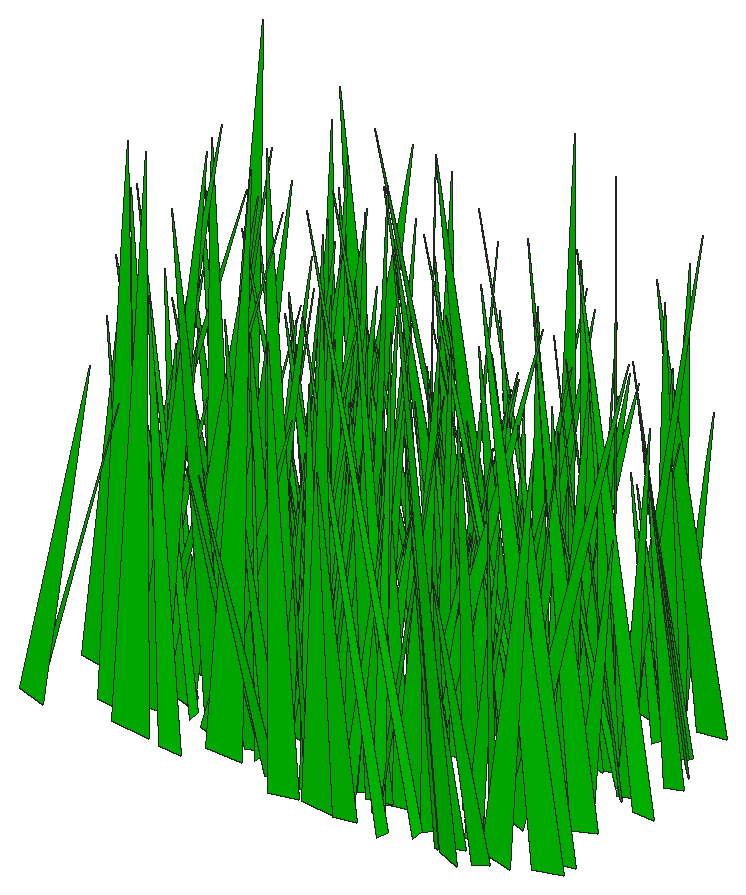
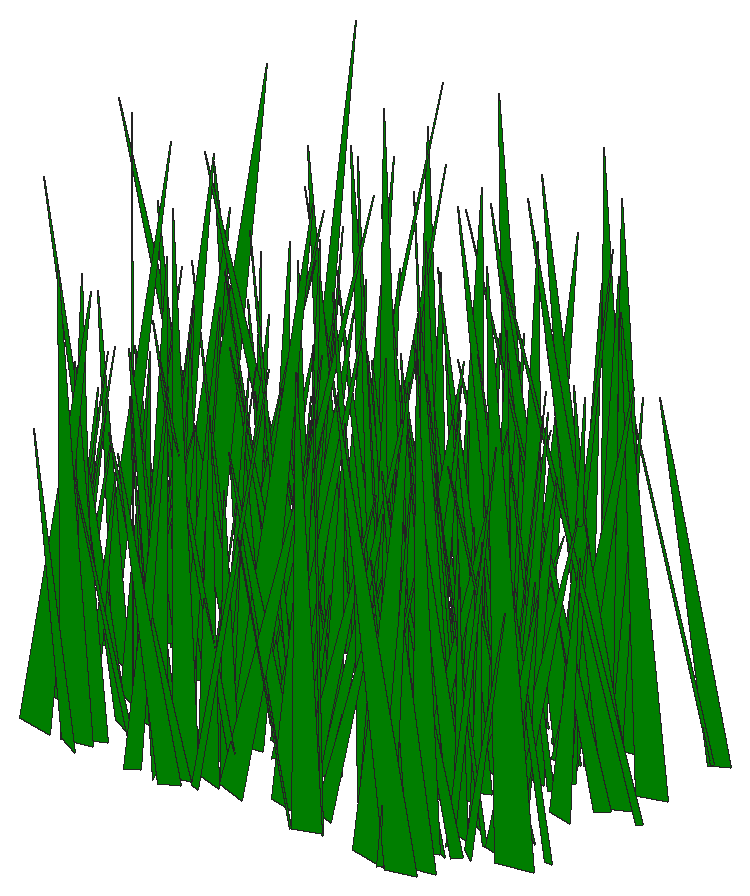
# SketchUp Ruby script. Lengths in inches.
U = 1.inch
M = Sketchup.active_model
def pt(a) = Geom::Point3d.new(a.map { |v| v * U })
def face(e, loops, mat)
  f = e.add_face(loops[0].map { |a| pt(a) })
  loops[1..].each { |l| e.add_face(l.map { |a| pt(a) }).erase! }
  f.material = f.back_material = mat if mat
  f
end
# faces: each face lists its corners as indices into pts; further lists are holes
def faces(e, pts, list, mat = nil) = list.each { |f| face(e, (f[0].is_a?(Array) ? f : [f]).map { |l| l.map { |i| pts[i] } }, mat) }
# xy, xz, yz: faces in a plane at the given z, y or x. An outline is a flat list of corners, or four numbers for a rectangle; further outlines are holes
def ring(l) = l.size == 4 ? [[l[0], l[1]], [l[2], l[1]], [l[2], l[3]], [l[0], l[3]]] : l.each_slice(2).to_a
def flat(e, list, mat, &to3) = list.each { |f| face(e, (f[0].is_a?(Array) ? f : [f]).map { |l| ring(l).map { |u, v| to3.(u, v) } }, mat) }
def xy(e, z, list, mat = nil) = flat(e, list, mat) { |x, y| [x, y, z] }
def xz(e, y, list, mat = nil) = flat(e, list, mat) { |x, z| [x, y, z] }
def yz(e, x, list, mat = nil) = flat(e, list, mat) { |y, z| [x, y, z] }
def lines(e, pts, list) = list.each { |a, b| e.add_line(pt(pts[a]), pt(pts[b])) }
# prism: a flat outline (further loops are holes) pulled along v
def prism(e, loops, v, mat = nil)
  f = face(e, loops, mat); d = Geom::Vector3d.new(v.map { |x| x * U })
  f.pushpull(f.normal.samedirection?(d) ? d.length : -d.length)
end
def box(e, o, s, mat = nil) = prism(e, [[o, [o[0] + s[0], o[1], o[2]], [o[0] + s[0], o[1] + s[1], o[2]], [o[0], o[1] + s[1], o[2]]]], [0, 0, s[2]], mat)
def at(x, y, z, deg = 0) = Geom::Transformation.translation(pt([x, y, z])) * Geom::Transformation.rotation(ORIGIN, Z_AXIS, deg.degrees)
def axes(o, x, y, z) = Geom::Transformation.new([*x, 0, *y, 0, *z, 0, *pt(o).to_a, 1])
def part(name) = M.definitions.add(name)
# library, detail: a bought-in or finely detailed component or shape, given as its bounding box
def library(name, o, s) = part(name).tap { |d| box(d.entities, o, s) }
def detail(e, o, s) = box(e.add_group.entities, o, s)
def put(e, d, t, mat = nil) = e.add_instance(d, t).tap { |i| i.material = mat if mat }
def group(e, t, mat = nil) = e.add_group.tap { |g| g.transformation = t; g.material = mat if mat }.entities
root = M.entities
M.materials.add("[Color G06]").color = [0, 204, 0]
c1 = part("fur_instance\#9")
p = [[0.8125,0,1.79],[0.67,-0.02,1.48],[0,-0.11,0],[0,0.11,0]]
faces(c1.entities,p,[[0,1,2,3]])
put(root,c1,axes([26.4,23.27,4.28],[-0.74577,0.42924,0.16576],[3.02431,0.09903,0.93683],[-0.58397,-0.03533,4.64003]),"[Color G06]")
put(root,c1,axes([25.05,18.42,4.28],[0.63249,-0.65402,1.81873],[-4.83005,-0.07148,0.79911],[0.38552,0.17738,7.02789]),"[Color G06]")
put(root,c1,axes([24.75,15.98,4.28],[1.15694,0.49328,0.89211],[3.55412,-0.14571,-1.04029],[0.48774,-0.10827,5.46438]),"[Color G06]")
put(root,c1,axes([26.29,20.73,4.28],[-0.22041,0.43199,0.02387],[3.06869,0.03014,0.63823],[-0.42484,-0.00643,4.59769]),"[Color G06]")
put(root,c1,axes([26.13,22.94,4.28],[-2.34809,-0.23299,0.75764],[-1.58293,0.33405,0.84245],[0.73687,-0.02483,4.22399]),"[Color G06]")
put(root,c1,axes([25.5625,23.53,4.28],[1.0567,-0.75927,3.56524],[-5.94438,-0.13239,0.69671],[0.04529,0.33887,8.26036]),"[Color G06]")
put(root,c1,axes([27.13,21.73,4.28],[-2.133,-0.40447,0.1356],[-2.89679,0.29581,-0.42214],[-0.17404,0.0335,5.36452]),"[Color G06]")
put(root,c1,axes([25.01,22.8,4.28],[4.72646,0.2099,1.45808],[1.58762,-0.66797,-0.44973],[-0.83481,-0.08195,7.39996]),"[Color G06]")
put(root,c1,axes([26.91,23.8,4.28],[-2.48961,-0.13509,1.03084],[-1.12689,0.33927,-0.97214],[0.37983,0.12113,3.8725]),"[Color G06]")
put(root,c1,axes([24.92,16.04,4.28],[3.51612,0.11611,0.22774],[0.84398,-0.48784,-0.53567],[-0.06488,-0.05355,5.3738]),"[Color G06]")
put(root,c1,axes([27.05,21.62,4.28],[-1.02199,-0.47937,1.50894],[-3.57415,0.12617,-0.80264],[-0.25033,0.1556,5.29972]),"[Color G06]")
put(root,c1,axes([27,21.7,4.28],[-3.25717,0.35501,2.09559],[2.77558,0.46707,0.54705],[0.86236,-0.1624,6.15443]),"[Color G06]")
put(root,c1,axes([27.27,22.03,4.28],[-4.4882,-0.06799,1.77196],[-0.37384,0.64522,0.7288],[1.22622,-0.05214,6.70794]),"[Color G06]")
put(root,c1,axes([25.62,19.78,4.28],[1.26546,0.38137,0.43753],[2.70664,-0.16467,-0.99861],[0.48937,-0.07544,4.39177]),"[Color G06]")
put(root,c1,axes([27.07,17.43,4.28],[-3.19454,-0.24212,1.99379],[-1.99642,0.45721,-0.76718],[0.89924,0.15493,5.37969]),"[Color G06]")
put(root,c1,axes([27.95,18.46,4.28],[-2.89977,0.47533,0.48212],[3.42219,0.40049,0.62015],[-0.10875,-0.0717,6.65977]),"[Color G06]")
put(root,c1,axes([24.42,19.73,4.28],[5.34845,0.24114,0.13319],[1.72825,-0.7409,-0.92994],[0.10717,-0.08637,8.34946]),"[Color G06]")
put(root,c1,axes([27.21,19.4,4.28],[-1.84379,-0.23386,1.66482],[-1.98406,0.24683,-0.92521],[0.34195,0.17119,3.6084]),"[Color G06]")
put(root,c1,axes([27.625,23.65,4.28],[-4.20743,0.09854,1.42356],[0.65174,0.60111,-0.47714],[0.99088,0.02305,6.35851]),"[Color G06]")
put(root,c1,axes([27.3,19.1875,4.28],[-3.20674,0.352,1.36352],[2.49266,0.46406,-0.66726],[0.99552,-0.02809,6.06289]),"[Color G06]")
put(root,c1,axes([27.33,17.78,4.28],[-3.59755,0.50257,1.75654],[3.61655,0.52274,-0.63547],[1.13623,-0.0726,7.58424]),"[Color G06]")
put(root,c1,axes([25.55,19.04,4.28],[3.42515,-0.42537,0.80037],[-3.09669,-0.47221,0.77246],[-0.05128,0.10354,6.81137]),"[Color G06]")
put(root,c1,axes([26.93,16.86,4.28],[-1.23965,0.81522,1.12811],[5.86982,0.18058,-0.58258],[0.54058,-0.09138,8.91273]),"[Color G06]")
put(root,c1,axes([25.3125,19.46,4.28],[4.76612,-0.52021,1.18159],[-3.79642,-0.66393,0.62771],[-0.35998,0.1143,9.02416]),"[Color G06]")
put(root,c1,axes([26.1,22.1,4.28],[3.69706,0.16509,0.09095],[1.16673,-0.51164,0.74681],[-0.20988,0.0638,5.75365]),"[Color G06]")
put(root,c1,axes([27.07,18.24,4.28],[2.22302,-0.48279,0.08933],[-3.43978,-0.30903,-0.6497],[-0.39795,-0.02578,6.11492]),"[Color G06]")
put(root,c1,axes([27.66,23.15,4.28],[1.30189,0.32159,1.09628],[2.34241,-0.19664,0.41254],[-0.60805,-0.06895,3.93652]),"[Color G06]")
put(root,c1,axes([27.85,22.33,4.28],[-2.25945,-0.1919,2.16686],[-1.82979,0.32139,-0.99221],[0.80481,0.19196,3.82747]),"[Color G06]")
put(root,c1,axes([28.26,25.58,4.28],[-3.47345,0.30399,1.18923],[2.10405,0.49678,-0.86016],[0.97893,0.01084,6.06838]),"[Color G06]")
put(root,c1,axes([26.86,23.15,4.28],[3.6365,-0.02019,1.00617],[-0.08995,-0.51417,-0.45894],[-0.6827,-0.03979,5.41993]),"[Color G06]")
put(root,c1,axes([27.3,25.2,4.28],[0.67891,0.57808,0.69955],[4.16154,-0.08918,-0.55572],[0.29386,-0.07259,6.25374]),"[Color G06]")
put(root,c1,axes([28.77,17.79,4.28],[-5.14485,0.07887,2.09535],[0.74235,0.73589,0.88946],[1.31695,-0.10669,7.68438]),"[Color G06]")
put(root,c1,axes([27.81,24.41,4.28],[3.19286,-0.4262,3.67293],[-3.68084,-0.47818,0.77329],[-1.35367,0.29497,6.56053]),"[Color G06]")
put(root,c1,axes([28.75,25.58,4.28],[-0.80445,0.6962,1.8653],[5.12572,0.09267,0.96458],[-0.45938,-0.18516,7.49629]),"[Color G06]")
put(root,c1,axes([27.34,19.78,4.28],[3.0252,0.14731,1.10939],[1.14425,-0.42804,-0.44094],[-0.59797,-0.07385,4.76876]),"[Color G06]")
put(root,c1,axes([28.36,19.55,4.28],[0.61584,0.72907,2.74837],[5.51261,-0.10724,0.50871],[-0.57273,-0.24825,7.85167]),"[Color G06]")
put(root,c1,axes([27.93,16.19,4.28],[-2.32148,0.72066,2.90787],[5.37717,0.362,-0.71684],[1.25697,-0.21762,8.43709]),"[Color G06]")
put(root,c1,axes([27.37,18.01,4.28],[3.71694,0.16434,1.67223],[1.38321,-0.52438,-0.94753],[-0.853,-0.1342,5.75027]),"[Color G06]")
put(root,c1,axes([29.36,19.87,4.28],[-1.86681,-0.31949,0.03301],[-2.23768,0.25337,-0.97569],[-0.4925,0.05983,4.30792]),"[Color G06]")
put(root,c1,axes([27.04,24.08,4.28],[3.31385,-0.19029,0.43767],[-1.38766,-0.46048,0.47035],[-0.1495,0.0562,5.3356]),"[Color G06]")
put(root,c1,axes([29.74,22.21,4.28],[-4.08264,0.20865,0.6781],[1.5461,0.56509,0.81896],[0.23302,-0.09373,6.44689]),"[Color G06]")
put(root,c1,axes([27.59,17.42,4.28],[3.32253,0.716,0.91072],[5.12861,-0.4692,0.58079],[-0.65824,-0.04161,9.12214]),"[Color G06]")
put(root,c1,axes([27.43,24.2,4.28],[2.84936,-0.05877,0.23266],[-0.38613,-0.39158,-0.79926],[-0.22968,-0.07076,4.23006]),"[Color G06]")
put(root,c1,axes([28.79,21.62,4.28],[-1.86066,0.33074,0.60389],[2.34538,0.26522,-0.54456],[0.5368,-0.01237,4.47249]),"[Color G06]")
put(root,c1,axes([28.01,20.68,4.28],[0.55032,-0.36921,0.01761],[-2.62203,-0.07576,0.5651],[0.36782,0.01232,4.00203]),"[Color G06]")
put(root,c1,axes([27.69,25.62,4.28],[1.023,0.69344,0.43741],[4.95055,-0.13689,-0.93351],[0.55428,-0.05725,7.53032]),"[Color G06]")
put(root,c1,axes([27.74,23.0625,4.28],[3.29325,-0.33143,1.33429],[-2.49573,-0.46003,0.63328],[-0.46608,0.12151,6.03683]),"[Color G06]")
put(root,c1,axes([28.36,23.77,4.28],[3.77664,-0.34019,2.91782],[-2.83355,-0.55286,0.78775],[-1.31679,0.214,6.67337]),"[Color G06]")
put(root,c1,axes([28.27,24.5625,4.28],[2.40695,-0.19485,1.26827],[-1.58258,-0.33053,0.87545],[-0.40999,0.13193,4.06647]),"[Color G06]")
put(root,c1,axes([26.67,18.6,4.28],[5.59212,0.20012,0.25968],[1.44387,-0.77797,-0.58167],[-0.07113,-0.0586,8.60904]),"[Color G06]")
put(root,c1,axes([29.52,17.875,4.28],[-3.19752,-0.62905,0.78295],[-4.4701,0.45172,0.91247],[0.80141,0.00978,8.21349]),"[Color G06]")
put(root,c1,axes([29.42,15.96,4.28],[-3.42101,0.41463,1.46619],[2.95457,0.49456,-0.66731],[1.0365,-0.04122,6.74141]),"[Color G06]")
put(root,c1,axes([30.01,24.375,4.28],[-3.25121,0.0824,0.64331],[0.6437,0.45236,0.61072],[0.34656,-0.06719,4.90088]),"[Color G06]")
put(root,c1,axes([27.97,18.25,4.28],[3.71945,0.5694,1.53485],[4.19806,-0.51616,-0.72787],[-0.32265,-0.15197,8.22292]),"[Color G06]")
put(root,c1,axes([28.74,20.99,4.28],[-0.85078,-0.48283,1.90775],[-3.56485,0.15475,0.94788],[0.9539,0.14768,5.24388]),"[Color G06]")
put(root,c1,axes([29.35,19.45,4.28],[-2.45848,0.40635,3.43893],[3.5618,0.36679,0.70905],[1.04866,-0.29316,5.65393]),"[Color G06]")
put(root,c1,axes([28.92,21.43,4.28],[3.95633,0.1568,1.6527],[1.08016,-0.57283,0.46719],[-1.14909,0.00138,6.12943]),"[Color G06]")
put(root,c1,axes([29.95,24.1875,4.28],[1.052,0.40935,1.6156],[3.02139,-0.17417,0.67478],[-0.81066,-0.11793,4.61151]),"[Color G06]")
put(root,c1,axes([29.85,18.6,4.28],[-1.88453,0.27138,0.98844],[1.93694,0.27634,-0.46675],[0.68793,-0.03463,4.0219]),"[Color G06]")
put(root,c1,axes([29.34,21.94,4.28],[0.58726,-0.65264,1.46217],[-4.7769,-0.07412,0.48507],[0.20737,0.14079,7.0331]),"[Color G06]")
put(root,c1,axes([30.56,21.15,4.28],[-1.98064,0.45114,1.64455],[3.41411,0.26884,0.71285],[0.14642,-0.16598,5.62449]),"[Color G06]")
put(root,c1,axes([29.02,18.9,4.28],[3.54411,0.64267,0.7797],[4.59685,-0.49889,0.56404],[-0.61771,-0.02534,8.67093]),"[Color G06]")
put(root,c1,axes([29.3,22.55,4.28],[1.25827,-0.45304,0.62976],[-3.27402,-0.17168,0.42517],[0.11554,0.06904,5.18971]),"[Color G06]")
put(root,c1,axes([29.4,21.07,4.28],[0.67413,0.67993,0.10104],[4.86721,-0.09323,-0.46531],[0.29919,-0.01527,7.34203]),"[Color G06]")
put(root,c1,axes([30.26,18.33,4.28],[-2.84836,-0.43528,1.16683],[-3.07562,0.41104,0.84366],[0.94556,0.02574,6.25912]),"[Color G06]")
put(root,c1,axes([31.07,17.35,4.28],[-1.91773,-0.31177,0.00303],[-2.21948,0.26542,-0.53331],[-0.26953,0.03261,4.36995]),"[Color G06]")
put(root,c1,axes([31.14,24.54,4.28],[-1.54449,-0.33272,0.32955],[-2.37456,0.20762,-0.77916],[-0.32117,0.065,4.17592]),"[Color G06]")
put(root,c1,axes([31.03,20.35,4.28],[-3.91535,0.078,1.4752],[0.39762,0.55752,-1.02905],[1.06256,0.07879,5.82093]),"[Color G06]")
put(root,c1,axes([30.875,18.96,4.28],[0.37624,0.79587,2.06586],[5.83839,-0.07145,0.78709],[-0.63115,-0.18654,8.51235]),"[Color G06]")
put(root,c1,axes([29.625,19.29,4.28],[3.78735,0.40354,1.67132],[3.02255,-0.53543,-0.44867],[-0.69958,-0.12865,7.10962]),"[Color G06]")
put(root,c1,axes([30.8,18.64,4.28],[0.73215,-0.60884,0.25969],[-4.33078,-0.10438,-0.83715],[-0.58135,0.01078,6.5635]),"[Color G06]")
put(root,c1,axes([30.51,23.54,4.28],[1.64288,0.40465,0.3521],[2.83435,-0.23092,0.94463],[-0.66534,0.01546,4.89351]),"[Color G06]")
put(root,c1,axes([30.87,19.2,4.28],[-2.7977,-0.17401,2.06353],[-1.54312,0.41121,-0.68998],[1.04027,0.14202,4.52613]),"[Color G06]")
put(root,c1,axes([30.61,25.28,4.28],[4.58409,-0.00772,2.77051],[0.14809,-0.68553,-0.76664],[-1.84862,-0.07405,6.80873]),"[Color G06]")
put(root,c1,axes([32.48,22.78,4.28],[-4.84411,0.20866,0.27643],[1.46293,0.67147,-0.95902],[0.36481,0.078,7.51649]),"[Color G06]")
put(root,c1,axes([29.72,17.29,4.28],[2.14078,0.44499,0.09364],[3.16148,-0.29418,-0.85166],[0.43876,-0.05145,5.67973]),"[Color G06]")
put(root,c1,axes([31.65,24.99,4.28],[-2.34039,0.19879,0.05679],[1.38755,0.31978,-0.85453],[0.3292,0.0654,4.00555]),"[Color G06]")
put(root,c1,axes([31.21,22.24,4.28],[-2.21436,-0.45508,2.89327],[-3.71044,0.32509,-0.46947],[0.79393,0.25007,5.87558]),"[Color G06]")
put(root,c1,axes([30.99,25.41,4.28],[-1.79137,0.59374,1.85382],[4.34064,0.27298,-0.67437],[0.90935,-0.1334,6.87098]),"[Color G06]")
put(root,c1,axes([30.4375,21.74,4.28],[0.16144,0.54475,2.38268],[4.16915,0.0136,-0.9881],[0.64849,-0.22303,5.75941]),"[Color G06]")
put(root,c1,axes([30.68,16.66,4.28],[3.18189,-0.67477,3.13501],[-5.19531,-0.45983,0.40901],[-0.90797,0.26642,8.64598]),"[Color G06]")
put(root,c1,axes([32.37,16.52,4.28],[-2.25234,-0.30552,0.00795],[-2.1765,0.31189,-0.54634],[-0.2511,0.03705,4.66431]),"[Color G06]")
put(root,c1,axes([32.37,19.5625,4.28],[-2.21424,0.49007,1.02794],[3.5773,0.29752,0.91864],[-0.16452,-0.12656,6.13979]),"[Color G06]")
put(root,c1,axes([32.57,23.39,4.28],[-2.57148,0.33224,0.27787],[2.38468,0.35422,0.64179],[-0.15691,-0.06147,5.19993]),"[Color G06]")
put(root,c1,axes([31.26,19.94,4.28],[3.03912,-0.33844,2.87158],[-2.85037,-0.4524,0.61352],[-1.20724,0.21615,5.78039]),"[Color G06]")
put(root,c1,axes([31.51,17.1,4.28],[2.82804,-0.14938,1.82601],[-0.93062,-0.42924,-0.8144],[-1.33202,-0.01727,4.44583]),"[Color G06]")
put(root,c1,axes([31.3,19.63,4.28],[-2.38322,-0.56698,2.76536],[-4.26427,0.37588,0.64394],[1.33104,0.18902,7.01435]),"[Color G06]")
put(root,c1,axes([32.1,17.03,4.28],[0.19945,-0.38177,0.70498],[-2.70347,-0.04185,-0.89511],[-0.63953,0.05786,4.00377]),"[Color G06]")
put(root,c1,axes([32.3,24.74,4.28],[1.2064,-0.48767,2.39437],[-3.69534,-0.21195,-0.80004],[-1.06838,0.18244,5.47089]),"[Color G06]")
put(root,c1,axes([32.53,19.05,4.28],[-2.08875,-0.33251,0.06435],[-2.36958,0.29025,0.47993],[0.2698,-0.02502,4.71339]),"[Color G06]")
put(root,c1,axes([31.55,21.72,4.28],[-4.15066,-0.34973,3.35294],[-2.45932,0.65433,1.03975],[2.29666,0.06863,7.17303]),"[Color G06]")
put(root,c1,axes([32.34,22.76,4.28],[-2.37959,0.44846,0.50869],[3.16921,0.3351,-0.82138],[0.64391,0.00796,5.92256]),"[Color G06]")
put(root,c1,axes([31.5625,22.13,4.28],[3.65184,0.45018,1.6072],[3.21831,-0.52838,0.6671],[-1.10503,-0.05115,7.25429]),"[Color G06]")
put(root,c1,axes([32.93,18.22,4.28],[-2.35819,0.17492,1.17324],[1.42434,0.32415,0.84332],[0.40122,-0.12265,3.902]),"[Color G06]")
put(root,c1,axes([31.43,25.5625,4.28],[2.84018,0.06126,0.50445],[0.48031,-0.39479,-0.53321],[-0.27607,-0.05664,4.2621]),"[Color G06]")
put(root,c1,axes([34.01,22.75,4.28],[-4.84535,0.29395,0.39332],[2.07304,0.67422,-0.83918],[0.46423,0.05733,7.85268]),"[Color G06]")
put(root,c1,axes([31.875,18.52,4.28],[1.88206,-0.40998,0.96908],[-3.0104,-0.2547,0.68138],[0.04396,0.11036,5.17268]),"[Color G06]")
put(root,c1,axes([32.08,17.47,4.28],[3.56157,-0.07027,1.45684],[-0.6196,-0.50979,0.55873],[-0.90565,0.07242,5.34693]),"[Color G06]")
put(root,c1,axes([33.86,25.01,4.28],[-1.25523,-0.50152,0.08168],[-3.5429,0.17099,-1.01154],[-0.62136,0.03818,5.60272]),"[Color G06]")
put(root,c1,axes([33.28,15.91,4.28],[0.15232,0.64931,1.0457],[4.68015,-0.03161,0.73174],[-0.51757,-0.09472,6.92451]),"[Color G06]")
put(root,c1,axes([33.11,18.08,4.28],[0.60124,-0.49103,0.93182],[-3.55393,-0.09184,-0.43737],[-0.3974,0.07844,5.32107]),"[Color G06]")
put(root,c1,axes([34.2,22.3,4.28],[-1.7898,-0.64934,0.36129],[-4.65491,0.24671,-0.57429],[-0.27262,0.05062,7.43388]),"[Color G06]")
put(root,c1,axes([32.9,16.39,4.28],[-1.87263,-0.3541,2.33199],[-2.69933,0.31044,0.57311],[1.2635,0.13841,4.68065]),"[Color G06]")
put(root,c1,axes([33.1,18.04,4.28],[-0.40227,0.44003,1.02854],[3.19352,0.06864,-0.58336],[0.48251,-0.08743,4.71852]),"[Color G06]")
put(root,c1,axes([32.29,24.26,4.28],[2.49778,-0.34276,0.20412],[-2.45379,-0.34445,0.62836],[0.19848,0.05508,5.19974]),"[Color G06]")
put(root,c1,axes([34.07,22.36,4.28],[-1.35779,-0.4355,1.34799],[-3.25069,0.18182,-0.56607],[-0.00194,0.13641,5.05813]),"[Color G06]")
put(root,c1,axes([34.74,25.41,4.28],[-4.62106,0.03699,1.22914],[0.37263,0.64822,0.88831],[0.77966,-0.09056,6.86062]),"[Color G06]")
put(root,c1,axes([33.93,16.17,4.28],[-2.67305,-0.13093,1.46976],[-1.09196,0.38694,-0.47622],[0.81015,0.08953,4.20751]),"[Color G06]")
put(root,c1,axes([33.83,16.48,4.28],[-1.76717,0.52618,1.19519],[3.81115,0.25708,-0.41426],[0.59401,-0.08407,6.21359]),"[Color G06]")
put(root,c1,axes([35.6875,21.92,4.28],[-5.77163,-0.32811,0.5497],[-2.33887,0.80626,0.42883],[0.44872,-0.01777,9.30553]),"[Color G06]")
put(root,c1,axes([32.96,19.5625,4.28],[4.21334,-0.15607,1.86919],[-1.34049,-0.59651,1.02813],[-1.00986,0.14066,6.4339]),"[Color G06]")
put(root,c1,axes([33.21,18.14,4.28],[3.27491,-0.53107,0.94542],[-3.79632,-0.46402,-0.56765],[-0.70151,0.03189,7.48553]),"[Color G06]")
put(root,c1,axes([33.23,17.625,4.28],[3.32897,0.09045,1.2459],[0.74153,-0.47385,-0.47391],[-0.75219,-0.06683,5.04676]),"[Color G06]")
put(root,c1,axes([33.1,19.13,4.28],[2.64944,-0.11781,0.37772],[-0.8716,-0.36679,0.51468],[-0.13388,0.05656,4.12423]),"[Color G06]")
put(root,c1,axes([35.04,22.9,4.28],[-3.10897,-0.74943,0.03712],[-5.35392,0.43222,0.78806],[0.46881,-0.03383,9.246]),"[Color G06]")
put(root,c1,axes([33.83,16.56,4.28],[4.37802,0.12791,2.571],[1.16539,-0.64444,-0.74989],[-1.56281,-0.12225,6.64314]),"[Color G06]")
put(root,c1,axes([34.07,18.0625,4.28],[-2.64566,-0.67981,2.89957],[-5.05371,0.41163,0.78606],[1.41091,0.19965,8.25266]),"[Color G06]")
put(root,c1,axes([33.76,19.37,4.28],[-0.07945,0.36947,1.345],[2.71737,0.04014,-0.90816],[0.66767,-0.11941,3.85621]),"[Color G06]")
put(root,c1,axes([34.17,24.64,4.28],[-0.80935,-0.41713,0.36272],[-2.93262,0.11737,0.88827],[0.63766,0.01035,4.54552]),"[Color G06]")
put(root,c1,axes([34.09,17.98,4.28],[-2.0214,-0.29826,2.20737],[-2.19005,0.33595,0.73476],[1.39996,0.09489,4.33665]),"[Color G06]")
put(root,c1,axes([34.69,24.92,4.28],[1.76167,0.45996,1.47717],[3.31721,-0.26822,0.75722],[-0.92357,-0.08602,5.53735]),"[Color G06]")
put(root,c1,axes([35.27,24.03,4.28],[-2.36546,0.31311,0.00689],[2.22454,0.32691,-0.65577],[0.30539,0.04394,4.8302]),"[Color G06]")
put(root,c1,axes([34.46,15.96,4.28],[-0.37187,-0.73953,1.58188],[-5.39588,0.06062,0.42229],[0.36131,0.14421,7.93452]),"[Color G06]")
put(root,c1,axes([35.19,23.67,4.28],[-3.44144,0.198,2.2952],[1.74598,0.49898,0.90302],[1.15151,-0.16484,5.4903]),"[Color G06]")
put(root,c1,axes([34.03,22.09,4.28],[4.74363,0.18345,2.20254],[1.52589,-0.67975,-0.8369],[-1.25466,-0.13311,7.30955]),"[Color G06]")
put(root,c1,axes([33.71,24.89,4.28],[4.02788,0.25741,0.51597],[1.81354,-0.56274,0.62617],[-0.48751,0.03331,6.59236]),"[Color G06]")
put(root,c1,axes([35.73,20.53,4.28],[-3.53784,0.25609,0.74118],[1.75206,0.49554,-0.98769],[0.74087,0.051,5.87508]),"[Color G06]")
put(root,c1,axes([35.33,15.93,4.28],[-0.38006,-0.50029,0.86478],[-3.62672,0.04706,-0.43293],[-0.23098,0.08429,5.37469]),"[Color G06]")
put(root,c1,axes([33.6875,21.97,4.28],[3.36968,0.2992,0.7046],[2.19556,-0.4628,-0.87883],[-0.07531,-0.10457,5.90553]),"[Color G06]")
put(root,c1,axes([35.42,17.27,4.28],[0.11676,-0.58245,0.94649],[-4.19693,-0.02609,-0.68793],[-0.48295,0.08592,6.2071]),"[Color G06]")
put(root,c1,axes([35.46,20.8125,4.28],[-2.83824,-0.22799,1.15044],[-1.59636,0.40998,0.53623],[0.84695,0.00872,4.866]),"[Color G06]")
put(root,c1,axes([35.73,20.79,4.28],[1.21779,-0.30153,2.24211],[-2.31881,-0.23195,-0.7701],[-1.24472,0.1371,3.62822]),"[Color G06]")
put(root,c1,axes([34.41,20.48,4.28],[0.68031,-0.48913,0.34055],[-3.48153,-0.08931,0.80091],[0.48425,0.0451,5.27973]),"[Color G06]")
put(root,c1,axes([35.8125,17.37,4.28],[-4.48144,0.29878,2.70657],[2.45692,0.64772,0.87323],[1.35421,-0.18641,7.37248]),"[Color G06]")
put(root,c1,axes([36.62,15.91,4.28],[-5.01431,0.13543,1.40874],[1.08356,0.70395,0.84115],[0.81091,-0.10319,7.58705]),"[Color G06]")
put(root,c1,axes([35.46,20.39,4.28],[0.50339,0.39066,0.44917],[2.79021,-0.07504,0.51188],[-0.39173,-0.03245,4.22319]),"[Color G06]")
put(root,c1,axes([34.89,16.59,4.28],[-2.15973,0.2402,2.34082],[1.66428,0.36761,-0.90335],[1.62802,-0.05714,4.02879]),"[Color G06]")
put(root,c1,axes([37.32,16.5,4.28],[-6.19557,0.06753,1.22263],[0.55521,0.86757,0.77971],[0.77167,-0.08201,9.2552]),"[Color G06]")
put(root,c1,axes([35.22,25.2,4.28],[-3.41588,-0.57147,3.25367],[-4.25064,0.53655,0.85744],[1.86174,0.17651,7.92742]),"[Color G06]")
put(root,c1,axes([34.98,21.59,4.28],[2.00919,0.45531,0.20944],[3.25176,-0.28081,0.44464],[-0.32676,0.00516,5.7126]),"[Color G06]")
put(root,c1,axes([36.09,24.37,4.28],[3.18462,0.31043,4.19241],[2.90402,-0.53016,-0.41788],[-2.09551,-0.26294,5.79225]),"[Color G06]")
put(root,c1,axes([34.9,17.55,4.28],[3.97067,-0.4833,1.39304],[-3.40937,-0.56849,-0.94939],[-1.12128,0.01708,7.81978]),"[Color G06]")
put(root,c1,axes([36.02,19.32,4.28],[-3.46202,0.14274,1.72629],[1.16574,0.50109,0.46239],[1.01146,-0.08894,5.37584]),"[Color G06]")
put(root,c1,axes([34.96,20.65,4.28],[3.02983,0.21291,0.53806],[1.44522,-0.42131,0.9727],[-0.61005,0.05933,4.97662]),"[Color G06]")
put(root,c1,axes([36.08,17.36,4.28],[-0.47063,0.54346,1.35594],[3.99559,0.05689,0.47862],[-0.21791,-0.13067,5.8476]),"[Color G06]")
put(root,c1,axes([35.74,19.46,4.28],[3.19647,0.3707,2.13829],[2.70917,-0.48043,0.52134],[-1.332,-0.08757,6.19169]),"[Color G06]")
put(root,c1,axes([36.72,22.51,4.28],[-3.75398,-0.09501,1.15286],[-0.6263,0.53371,0.49711],[0.81667,-0.02742,5.68055]),"[Color G06]")
put(root,c1,axes([36.64,25.67,4.28],[-3.52857,0.29763,1.2323],[2.12228,0.5047,-0.42854],[0.85513,-0.02447,6.14851]),"[Color G06]")
put(root,c1,axes([35.07,19.43,4.28],[2.71539,0.07086,0.51872],[0.57774,-0.36896,-0.96542],[-0.21193,-0.09789,4.01436]),"[Color G06]")
put(root,c1,axes([36.47,21.51,4.28],[-0.26482,-0.58075,1.13959],[-4.21846,0.02709,-0.60377],[-0.36168,0.10925,6.20775]),"[Color G06]")
put(root,c1,axes([35.88,16.65,4.28],[-4.28438,0.22328,3.04618],[1.49579,0.66141,-0.86975],[2.1167,-0.01547,6.78033]),"[Color G06]")
put(root,c1,axes([35.36,25.72,4.28],[0.47319,0.48756,0.3161],[3.44906,-0.05966,-0.96213],[0.61119,-0.0408,5.18475]),"[Color G06]")
put(root,c1,axes([37.91,20.49,4.28],[-5.32174,0.18608,0.7773],[1.3704,0.74269,0.53391],[0.41612,-0.06614,8.18256]),"[Color G06]")
put(root,c1,axes([35.02,23.89,4.28],[3.50847,0.36596,0.98479],[2.68422,-0.4897,-0.45621],[-0.34146,-0.08937,6.53244]),"[Color G06]")
put(root,c1,axes([37.16,20.78,4.28],[-1.8253,0.42199,0.48083],[3.03831,0.24972,0.58804],[-0.17317,-0.06663,5.24907]),"[Color G06]")
put(root,c1,axes([35.93,25.63,4.28],[3.62986,0.01375,1.8416],[-0.01149,-0.53261,0.50732],[-1.23607,0.04532,5.40333]),"[Color G06]")
put(root,c1,axes([35.53,18.84,4.28],[0.93268,0.38093,0.3372],[2.70698,-0.12278,-0.79148],[0.43103,-0.0532,4.24103]),"[Color G06]")
put(root,c1,axes([35.27,25.3125,4.28],[2.09574,0.40835,0.18291],[2.91498,-0.2882,-0.69143],[0.30579,-0.05133,5.33748]),"[Color G06]")
put(root,c1,axes([36.83,23.22,4.28],[0.16578,0.46555,0.70219],[3.34779,-0.03049,0.55664],[-0.39879,-0.06243,4.96477]),"[Color G06]")
put(root,c1,axes([36.78,18.26,4.28],[3.57136,0.16762,3.269],[1.71697,-0.55144,-0.94184],[-1.81135,-0.19222,5.55258]),"[Color G06]")
put(root,c1,axes([35.83,16.6875,4.28],[4.46304,0.17627,1.12327],[1.16334,-0.62803,0.99636],[-0.89965,0.06235,6.86076]),"[Color G06]")
put(root,c1,axes([36.29,17.375,4.28],[-1.74938,-0.59957,3.00557],[-4.51974,0.30171,1.03764],[1.45018,0.21706,6.85964]),"[Color G06]")
put(root,c1,axes([38.66,19.73,4.28],[-4.83613,0.04179,0.32792],[0.28575,0.67386,-0.45268],[0.23731,0.04031,7.22765]),"[Color G06]")
put(root,c1,axes([35.28,19.36,4.28],[4.80618,-0.35351,0.36321],[-2.54494,-0.66391,0.99207],[0.09666,0.09764,8.06042]),"[Color G06]")
put(root,c1,axes([37.66,23.56,4.28],[-2.2654,0.52351,3.06165],[4.20449,0.3318,0.43191],[0.78296,-0.26703,6.53915]),"[Color G06]")
put(root,c1,axes([37.43,16.82,4.28],[1.44143,-0.32235,0.22863],[-2.23349,-0.20003,-0.94386],[-0.61546,-0.02906,3.96069]),"[Color G06]")
put(root,c1,axes([37.55,22.33,4.28],[1.95223,0.27055,1.09183],[1.87507,-0.29011,0.76904],[-0.8843,-0.01789,4.04106]),"[Color G06]")
put(root,c1,axes([38.18,16.23,4.28],[-3.81973,-0.12197,1.83504],[-0.99676,0.55423,-0.40297],[1.13092,0.07653,5.84275]),"[Color G06]")
put(root,c1,axes([37.3,23.35,4.28],[2.42897,0.26338,0.78893],[1.83005,-0.34652,0.70367],[-0.70503,0.00793,4.54451]),"[Color G06]")
put(root,c1,axes([37.875,18.18,4.28],[-2.19168,-0.50683,0.95451],[-3.58783,0.31689,0.92722],[0.8635,0.03027,6.27522]),"[Color G06]")
put(root,c1,axes([38.76,16,4.28],[-5.19678,-0.43742,2.11241],[-3.12461,0.74948,0.65729],[1.4402,0.04767,9.04838]),"[Color G06]")
put(root,c1,axes([38.54,16.53,4.28],[-0.47681,-0.5143,0.03028],[-3.66146,0.06566,-0.67267],[-0.44379,0.01083,5.5173]),"[Color G06]")
put(root,c1,axes([37.46,23.23,4.28],[1.31188,0.43846,2.248],[3.48355,-0.15737,-1.01502],[0.11759,-0.22955,4.98982]),"[Color G06]")
put(root,c1,axes([38.95,22.17,4.28],[-4.22616,0.04617,1.45064],[0.25871,0.60338,-0.5223],[0.99235,0.0393,6.3141]),"[Color G06]")
put(root,c1,axes([37.1875,24.95,4.28],[2.90912,0.19293,0.08199],[1.37245,-0.40413,0.46668],[-0.18344,0.03606,4.79191]),"[Color G06]")
put(root,c1,axes([38.375,20.98,4.28],[-1.89759,0.45419,0.48349],[3.18675,0.26827,-1.01119],[0.74695,0.00932,5.54238]),"[Color G06]")
put(root,c1,axes([39.05,22.87,4.28],[2.2239,0.30217,2.39236],[2.28599,-0.36481,0.54639],[-1.42552,-0.11361,4.60845]),"[Color G06]")
put(root,c1,axes([39.125,24.31,4.28],[-2.31371,0.15643,1.39873],[1.33206,0.32627,0.73022],[0.59993,-0.12114,3.77302]),"[Color G06]")
put(root,c1,axes([38.29,25.11,4.28],[-0.58993,-0.50692,1.54225],[-3.70234,0.1067,0.86526],[0.75671,0.12684,5.4358]),"[Color G06]")
put(root,c1,axes([39.88,21.8,4.28],[-2.86016,0.10842,0.25709],[0.79353,0.39552,0.5588],[0.06642,-0.05664,4.39446]),"[Color G06]")
put(root,c1,axes([37.9375,17.84,4.28],[3.45974,0.18186,0.77392],[1.26737,-0.48745,0.5029],[-0.60237,0.01897,5.5031]),"[Color G06]")
put(root,c1,axes([38.77,22.97,4.28],[5.48883,0.03786,3.64774],[0.50229,-0.83305,-0.69501],[-2.40379,-0.08762,8.18404]),"[Color G06]")
put(root,c1,axes([39.14,22.28,4.28],[0.90327,0.48669,1.12248],[3.49535,-0.14254,0.81682],[-0.72645,-0.08071,5.32587]),"[Color G06]")
put(root,c1,axes([39.65,16.26,4.28],[-0.9578,-0.37767,0.64843],[-2.71458,0.12134,-0.83843],[-0.39301,0.08232,4.21085]),"[Color G06]")
put(root,c1,axes([38.65,17.1875,4.28],[1.9228,0.3869,0.63609],[2.76405,-0.27351,0.44678],[-0.48912,-0.02466,5.02538]),"[Color G06]")
put(root,c1,axes([38.63,25.5,4.28],[0.43331,0.58387,3.45091],[4.7767,-0.03837,-0.59408],[0.21434,-0.32534,6.26319]),"[Color G06]")
put(root,c1,axes([38.74,25.72,4.28],[2.46172,0.3392,0.31491],[2.35916,-0.3412,1.02318],[-0.62899,0.04779,5.07016]),"[Color G06]")
put(root,c1,axes([38.49,19.02,4.28],[3.69966,0.09539,1.43107],[0.86482,-0.51913,-1.01893],[-0.79805,-0.12034,5.53006]),"[Color G06]")
put(root,c1,axes([40.05,25.47,4.28],[-1.25234,-0.64955,0.65494],[-4.66923,0.1695,-0.63199],[-0.2967,0.07416,7.18131]),"[Color G06]")
put(root,c1,axes([39.2,24.65,4.28],[-0.78154,-0.62714,1.37088],[-4.56825,0.1189,0.43075],[0.44635,0.11875,6.80885]),"[Color G06]")
put(root,c1,axes([39.32,17.2,4.28],[2.98927,0.17731,2.78625],[1.78745,-0.44941,-0.99827],[-1.3774,-0.1984,4.75134]),"[Color G06]")
put(root,c1,axes([40.33,21.29,4.28],[-4.30964,-0.00322,1.31901],[-0.10618,0.61067,-0.60382],[0.87642,0.05816,6.4128]),"[Color G06]")
put(root,c1,axes([40.34,24.05,4.28],[-3.79479,-0.12156,1.21174],[-0.97782,0.5337,-0.69002],[0.67903,0.08922,5.77826]),"[Color G06]")
put(root,c1,axes([38.25,24.07,4.28],[4.91572,0.35889,1.18889],[2.53765,-0.69439,0.64223],[-0.90396,0.00233,8.26808]),"[Color G06]")
put(root,c1,axes([40.24,24.07,4.28],[1.00891,0.36551,2.40876],[2.80633,-0.2063,0.9704],[-1.26188,-0.16656,4.08397]),"[Color G06]")
put(root,c1,axes([39.83,19.89,4.28],[2.83483,0.1484,2.88913],[1.57382,-0.44357,-0.83216],[-1.54674,-0.17936,4.44839]),"[Color G06]")
put(root,c1,axes([40.48,23.34,4.28],[-2.36284,0.25856,0.06174],[1.83772,0.32765,-0.52763],[0.25024,0.0352,4.45787]),"[Color G06]")
put(root,c1,axes([39.21,20.1,4.28],[2.28407,0.48274,2.83251],[3.92427,-0.31027,-0.9942],[-0.41974,-0.2739,6.11841]),"[Color G06]")
put(root,c1,axes([40.65,19.35,4.28],[2.69029,-0.46953,4.25444],[-3.81749,-0.48072,-0.70223],[-2.2062,0.25925,6.40306]),"[Color G06]")
put(root,c1,axes([41.26,17.0625,4.28],[-3.67708,0.63342,1.37162],[4.62546,0.51169,0.55362],[0.28482,-0.13217,8.71702]),"[Color G06]")
put(root,c1,axes([40.8,23.5,4.28],[-3.54068,-0.13795,0.99258],[-0.87986,0.4985,0.94797],[0.80348,-0.06202,5.41209]),"[Color G06]")
put(root,c1,axes([41.34,20.98,4.28],[-4.98732,0.37434,1.19875],[2.65817,0.70437,-0.56407],[0.88535,-0.00609,8.4463]),"[Color G06]")
put(root,c1,axes([41.29,17.58,4.28],[-1.70453,0.59244,0.29005],[4.24736,0.23563,0.46801],[-0.21879,-0.04133,6.82574]),"[Color G06]")
put(root,c1,axes([39.81,16.7,4.28],[0.65131,0.57286,2.15669],[4.3378,-0.06772,-0.85981],[0.37763,-0.21013,6.15686]),"[Color G06]")
put(root,c1,axes([40.34,21.5,4.28],[2.49001,0.42651,0.89236],[3.00426,-0.35686,0.86805],[-0.82839,-0.01215,5.8304]),"[Color G06]")
put(root,c1,axes([41.05,22.62,4.28],[0.48564,-0.37535,1.95371],[-2.91372,-0.10137,-0.61945],[-0.68148,0.16594,4.04074]),"[Color G06]")
put(root,c1,axes([40.21,19.87,4.28],[0.30843,0.40967,1.00377],[2.99356,-0.03079,-0.61095],[0.34747,-0.09835,4.37252]),"[Color G06]")
put(root,c1,axes([38.9,18.59,4.28],[4.5153,0.43604,0.45636],[3.14182,-0.62647,-0.67626],[0.00783,-0.07611,8.1808]),"[Color G06]")
